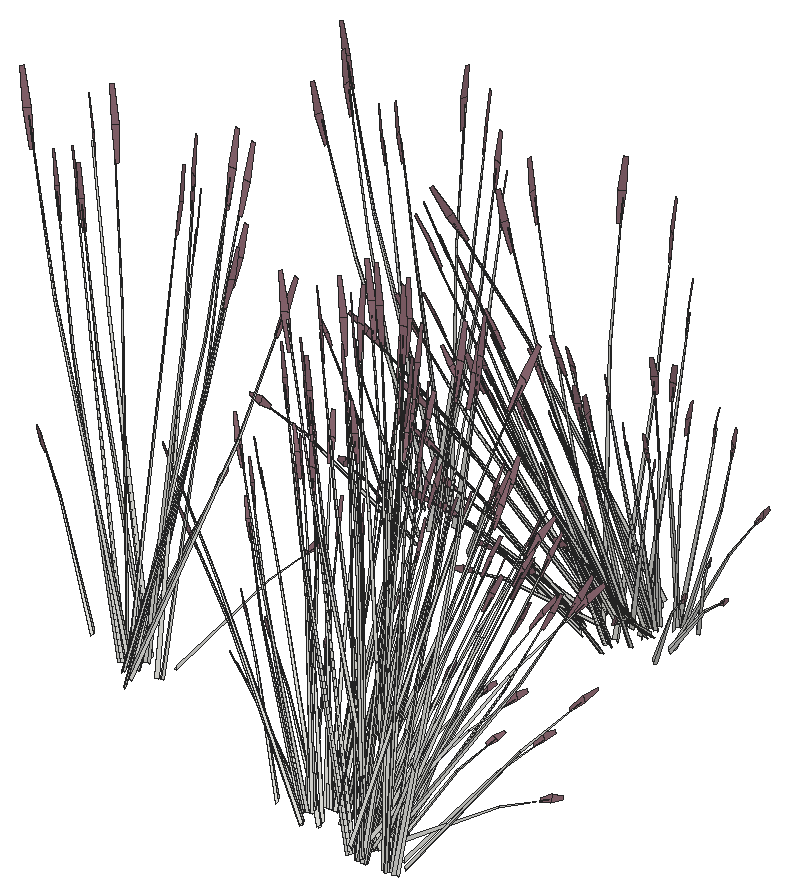
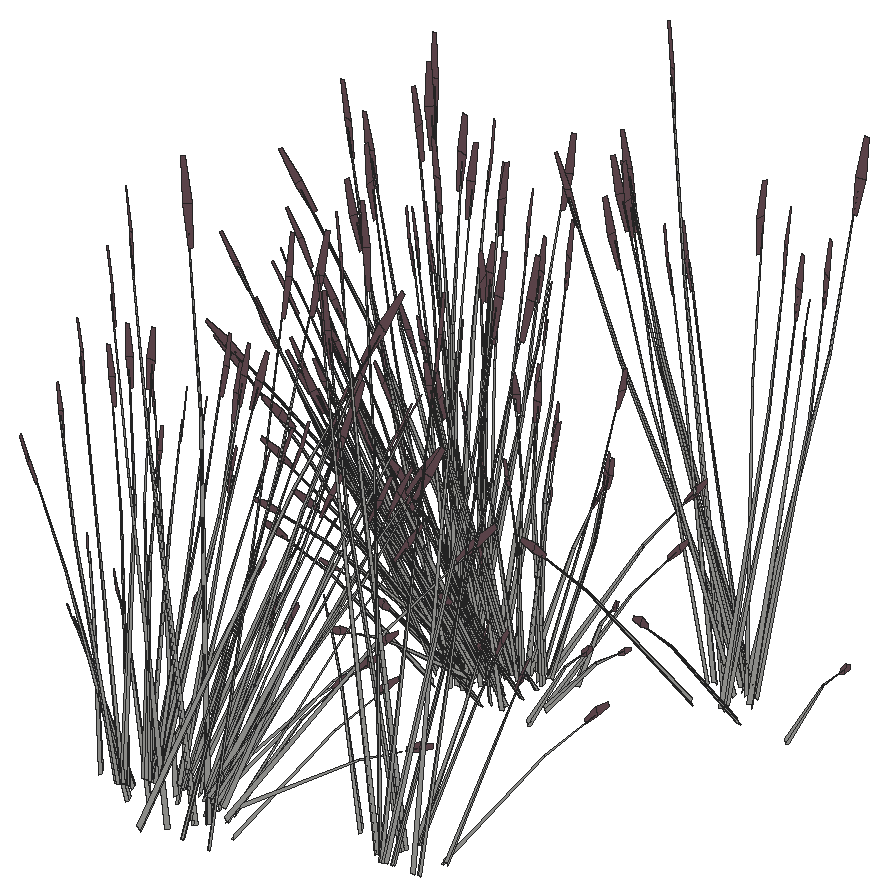
# SketchUp Ruby script. Lengths in inches.
U = 1.inch
M = Sketchup.active_model
def pt(a) = Geom::Point3d.new(a.map { |v| v * U })
def face(e, loops, mat)
  f = e.add_face(loops[0].map { |a| pt(a) })
  loops[1..].each { |l| e.add_face(l.map { |a| pt(a) }).erase! }
  f.material = f.back_material = mat if mat
  f
end
# faces: each face lists its corners as indices into pts; further lists are holes
def faces(e, pts, list, mat = nil) = list.each { |f| face(e, (f[0].is_a?(Array) ? f : [f]).map { |l| l.map { |i| pts[i] } }, mat) }
# xy, xz, yz: faces in a plane at the given z, y or x. An outline is a flat list of corners, or four numbers for a rectangle; further outlines are holes
def ring(l) = l.size == 4 ? [[l[0], l[1]], [l[2], l[1]], [l[2], l[3]], [l[0], l[3]]] : l.each_slice(2).to_a
def flat(e, list, mat, &to3) = list.each { |f| face(e, (f[0].is_a?(Array) ? f : [f]).map { |l| ring(l).map { |u, v| to3.(u, v) } }, mat) }
def xy(e, z, list, mat = nil) = flat(e, list, mat) { |x, y| [x, y, z] }
def xz(e, y, list, mat = nil) = flat(e, list, mat) { |x, z| [x, y, z] }
def yz(e, x, list, mat = nil) = flat(e, list, mat) { |y, z| [x, y, z] }
def lines(e, pts, list) = list.each { |a, b| e.add_line(pt(pts[a]), pt(pts[b])) }
# prism: a flat outline (further loops are holes) pulled along v
def prism(e, loops, v, mat = nil)
  f = face(e, loops, mat); d = Geom::Vector3d.new(v.map { |x| x * U })
  f.pushpull(f.normal.samedirection?(d) ? d.length : -d.length)
end
def box(e, o, s, mat = nil) = prism(e, [[o, [o[0] + s[0], o[1], o[2]], [o[0] + s[0], o[1] + s[1], o[2]], [o[0], o[1] + s[1], o[2]]]], [0, 0, s[2]], mat)
def at(x, y, z, deg = 0) = Geom::Transformation.translation(pt([x, y, z])) * Geom::Transformation.rotation(ORIGIN, Z_AXIS, deg.degrees)
def axes(o, x, y, z) = Geom::Transformation.new([*x, 0, *y, 0, *z, 0, *pt(o).to_a, 1])
def part(name) = M.definitions.add(name)
# library, detail: a bought-in or finely detailed component or shape, given as its bounding box
def library(name, o, s) = part(name).tap { |d| box(d.entities, o, s) }
def detail(e, o, s) = box(e.add_group.entities, o, s)
def put(e, d, t, mat = nil) = e.add_instance(d, t).tap { |i| i.material = mat if mat }
def group(e, t, mat = nil) = e.add_group.tap { |g| g.transformation = t; g.material = mat if mat }.entities
root = M.entities
M.materials.add("LightPink_Translucent").color = [144, 107, 117]
c1 = part("blade")
p = [[2.15,0.21,22],[0,0.17,0],[0.09,0.45,0],[2.18,0.31,22],[2.29,0.31,22],[0.38,0.45,0],
  [2.48,0.24,33],[2.49,0.24,33],[2.48,0.22,33]]
faces(c1.entities,p,[[0,1,2,3],[4,5,2,3],[6,3,4,7],[8,0,3,6]])
c2 = part("seeds")
p = [[0.3,-0.1,1.38],[-0.01,-0.03,1.59],[-0.01,-0.03,0.03],[0.14,-0.07,-0.07],[0.29,-0.03,3],[0.15,0.01,3.11]]
faces(c2.entities,p,[[0,1,2,3],[1,0,4,5]],"LightPink_Translucent")
c3 = part("blade with seeds")
put(c3.entities,c1,at(0,0,0))
put(c3.entities,c2,axes([2.4,0.25,30.99],[1.5799,-0.05474,1.17369],[-0.12525,1.92788,0.29478],[-0.07173,-0.02425,1.56792]))
put(root,c3,axes([79.25,512.875,37.29],[0.06562,-1.05324,-0.1216],[1.2424,0.02879,-0.67495],[0.4785,0.07316,1.02557]))
put(root,c3,axes([80.38,510.0625,34.73],[0,-1.03566,0.49651],[1.37109,0,0],[0,0.23588,1.57504]))
put(root,c3,axes([49.21,509.61,44.03],[0.28787,0.90242,-0.30978],[-1.14332,0.25625,0.30978],[0.23049,0.10406,1.38974]))
put(root,c3,axes([76.94,510.84,34.97],[1.33077,-0.06393,0.44739],[0.12035,1.06125,-0.21531],[-0.23824,0.10756,1.43643]))
put(root,c3,axes([77.77,509.76,34.87],[1.1418,-0.30203,0.1448],[0.39985,0.86246,-0.41347],[0,0.18981,1.26744]))
put(root,c3,axes([79.06,512.46,37.31],[-0.69728,-0.64842,0.35414],[0.79619,-0.61382,-0.4572],[0.40453,0.09339,0.87481]))
put(root,c3,axes([75.76,511.35,34.47],[-1.33077,0.06393,-0.44739],[-0.12035,-1.06125,0.21531],[-0.23824,0.10756,1.43643]))
put(root,c3,axes([82.02,511.86,34.85],[-0.29514,-0.25472,1.43002],[0.38401,-0.84262,-0.30754],[0.59714,0.11414,0.61141]))
put(root,c3,axes([47.17,514.54,44.18],[1.2866,-0.3514,-0.19198],[0.45209,1.01223,0.00008],[0.14202,-0.03884,1.73897]))
put(root,c3,axes([76.74,512.78,34.46],[1.23546,0.46496,0],[-0.59459,0.96613,0],[0,0,1.74954]))
put(root,c3,axes([47.86,511.2,44.06],[1.27479,0.1698,-0.62353],[-0.26901,1.04736,-0.16365],[0.38043,0.12691,1.37633]))
put(root,c3,axes([80.33,512.24,36.97],[0.26289,-0.01751,1.74944],[0.72108,-0.8046,-0.27667],[0.46761,0.10621,0.14031]))
put(root,c3,axes([77.23,513.8125,34.45],[-0.75665,-1.04141,-0.05142],[1.28187,-0.57875,0.51607],[-0.31588,0.09915,1.6363]))
put(root,c3,axes([76.97,511.29,34.87],[0.90538,0.62224,0.1448],[-0.75521,0.70202,-0.41347],[-0.21021,0.09491,1.26744]))
put(root,c3,axes([69.82,511.46,36.99],[-0.30393,-0.95317,0.48003],[1.19224,-0.16542,0.3958],[-0.35138,0.22417,0.9933]))
put(root,c3,axes([69.58,511.27,36.98],[-0.8413,-0.43556,0.0643],[0.48981,-0.62025,0.50621],[-0.26973,0.20053,0.77189]))
put(root,c3,axes([69.96,510.125,36.13],[0.42521,-0.21906,1.71376],[0.35798,1.01226,0.13857],[-0.66754,0.22878,0.73262]))
put(root,c3,axes([46.42,513.84,44.46],[-1.19666,-0.83357,-0.25192],[1.00694,-0.93603,0.5513],[-0.32224,0.09751,1.68216]))
put(root,c3,axes([79.31,512.37,37.24],[1.22504,0.02494,-0.71045],[-0.08228,1.05005,0.08574],[0.51899,0.11081,1.00501]))
put(root,c3,axes([77.93,513.21,34.73],[1.14694,-0.51783,0.49651],[0.68554,0.92854,0],[-0.26122,0.11794,1.57504]))
put(root,c3,axes([47.2,511.53,44.21],[0.73619,0.86927,-0.44739],[-1.11511,0.61213,0.21531],[0.23824,0.10756,1.43643]))
put(root,c3,axes([76.3,512.39,34.55],[0.53281,1.18979,-0.06012],[-1.52239,0.41691,0],[0.01861,0.04155,1.72173]))
put(root,c3,axes([76.89,513.68,34.28],[-1.14332,-0.25625,-0.30978],[0.28787,-0.90242,0.30978],[-0.23049,0.10406,1.38974]))
put(root,c3,axes([68.64,511.85,34.85],[0.42589,0.08502,1.43002],[0.2745,0.86839,-0.30754],[-0.57851,0.16255,0.61141]))
put(root,c3,axes([70.55,511.14,37.31],[1.06674,-0.14801,0.35414],[0.28168,0.84611,-0.4572],[-0.30569,0.22726,0.87481]))
put(root,c3,axes([81.31,510.24,34.63],[1.53239,0,0],[0,1.1575,-0.51607],[0,0.26363,1.63711]))
put(root,c3,axes([66.4375,510.76,36.96],[0.1564,0.02778,1.77383],[0.48382,0.91506,-0.16761],[-0.32016,0.24017,0.31391]))
put(root,c3,axes([80.7,510.83,34.45],[-1.53164,-0.00828,-0.04976],[0,-1.1575,0.49943],[-0.04813,0.2635,1.58352]))
put(root,c3,axes([77.38,509.83,34.92],[1.38012,0.49416,-0.29095],[-0.66454,1.04299,-0.50002],[0.04337,0.25608,1.59708]))
put(root,c3,axes([45.8125,513.66,44.21],[-1.33077,0.06393,-0.44739],[-0.12035,-1.06125,0.21531],[-0.23824,0.10756,1.43643]))
put(root,c3,axes([67.75,513.67,35.02],[0.51072,-0.46938,1.1486],[0.20153,0.74307,0.84392],[-0.36908,0.13305,0.25299]))
put(root,c3,axes([80.05,512.8,36.78],[0.69728,0.64842,-0.35414],[-0.79619,0.61382,0.4572],[0.40453,0.09339,0.87481]))
put(root,c3,axes([80.38,511,34.28],[-0.85545,0.64616,-0.30978],[-0.85545,-0.64616,0.30978],[0,0.20813,1.38974]))
put(root,c3,axes([76.69,511.06,34.92],[0.1428,1.18174,-0.29095],[-1.48733,0.07145,-0.50002],[-0.26191,0.15741,1.59708]))
put(root,c3,axes([79.6875,513.05,36.98],[-0.06171,0.78753,0.0643],[-0.9318,-0.02159,0.50621],[0.35694,0.08241,0.77189]))
put(root,c3,axes([77.24,510.6,34.47],[-0.59459,0.93321,-0.44739],[-1.23546,-0.44912,0.21531],[0,0.21512,1.43643]))
put(root,c3,axes([69.68,511.64,36.78],[-1.06674,0.14801,-0.35414],[-0.28168,-0.84611,0.4572],[-0.30569,0.22726,0.87481]))
put(root,c3,axes([79.77,512.8,36.99],[-0.90362,0.68241,0.48003],[-0.77932,-0.72471,0.3958],[0.42395,0.12588,0.9933]))
put(root,c3,axes([68.125,513.54,37.9],[1.08141,0.27645,-0.06488],[-0.33265,0.85086,-0.29416],[-0.17688,0.12919,0.97024]))
put(root,c3,axes([75.8,511.97,34.3125],[-0.82544,0.77843,-0.62353],[-1.0254,-0.70586,-0.16365],[-0.33076,0.19418,1.37633]))
put(root,c3,axes([76.9,513.59,37.31],[-0.18927,-0.83419,0.35414],[1.08199,-0.22027,-0.4572],[0.29062,0.23905,0.87481]))
put(root,c3,axes([77.27,513.28,34.58],[1.53422,0.33662,0.30756],[-0.38383,1.20322,-0.36492],[-0.25393,0.15059,1.64885]))
put(root,c3,axes([77.16,514.09,34.27],[-1.14694,0.51783,-0.49651],[-0.68554,-0.92854,0],[-0.26122,0.11794,1.57504]))
put(root,c3,axes([80.97,511.02,34.27],[0,1.03566,-0.49651],[-1.37109,0,0],[0,0.23588,1.57504]))
put(root,c3,axes([77.54,511.14,36.13],[-0.45521,-0.17844,1.71376],[0.94204,-0.74856,0.13857],[0.58713,0.33769,0.73262]))
put(root,c3,axes([77.63,508.79,36.73],[-1.05895,-0.53811,1.38283],[1.11816,-0.83781,0.59665],[0.34166,0.5049,1.33663]))
put(root,c3,axes([70,511.0625,37.29],[1.1336,0.57106,-0.1216],[-0.65308,0.827,-0.67495],[-0.32027,0.28747,1.02557]))
put(root,c3,axes([46.94,515.99,44.03],[-1.14332,-0.25625,-0.30978],[0.28787,-0.90242,0.30978],[-0.23049,0.10406,1.38974]))
put(root,c3,axes([79.23,513.17,35.02],[-0.69001,-0.29779,1.1486],[0.89096,-0.30257,0.84392],[0.24031,0.2563,0.25299]))
put(root,c3,axes([76.8,514.02,37.29],[0.73026,-0.88648,-0.1216],[1.05755,0.51071,-0.67495],[0.36761,0.25045,1.02557]))
put(root,c3,axes([71.52,510.81,36.13],[0.30609,-0.31822,1.71376],[0.77286,0.85893,0.13857],[-0.53009,0.39116,0.73262]))
put(root,c3,axes([47.4375,512.13,44.67],[1.38012,0.49416,-0.29095],[-0.66454,1.04299,-0.50002],[0.04337,0.25608,1.59708]))
put(root,c3,axes([70.56,511.74,36.94],[0.31482,0.94565,-0.51099],[-1.19224,0.16542,-0.3958],[-0.34166,0.254,0.97773]))
put(root,c3,axes([50.43,513.31,44.03],[-0.85545,0.64616,-0.30978],[-0.85545,-0.64616,0.30978],[0,0.20813,1.38974]))
put(root,c3,axes([71.99,512.83,37.31],[0.82919,-0.54528,0.35414],[0.78493,0.62262,-0.4572],[-0.11943,0.31634,0.87481]))
put(root,c3,axes([78.2,513.93,34.63],[0.7662,1.03778,0],[-1.28187,0.57875,-0.51607],[-0.29196,0.13181,1.63711]))
put(root,c3,axes([46.75,513.37,44.67],[0.1428,1.18174,-0.29095],[-1.48733,0.07145,-0.50002],[-0.26191,0.15741,1.59708]))
put(root,c3,axes([75.85,514.76,36.96],[0.00363,-0.12539,1.77383],[1.0502,-0.55319,-0.16761],[0.36479,0.19745,0.31391]))
put(root,c3,axes([47.29,512.91,44.21],[-0.59459,0.93321,-0.44739],[-1.23546,-0.44912,0.21531],[0,0.21512,1.43643]))
put(root,c3,axes([79.42,514.28,33.75],[0.08928,-0.14952,1.76342],[1.12407,-0.44035,-0.26939],[0.34078,0.22791,0.30037]))
put(root,c3,axes([77.55,509.82,35.1],[-0.03348,-0.97511,1.41272],[1.51511,0.25277,0.59816],[-0.35835,0.53357,1.3335]))
put(root,c3,axes([77.94,510.88,34.35],[0.44936,0.94823,-0.69212],[-1.29441,0.3415,-0.18165],[0.04967,0.32109,1.52773]))
put(root,c3,axes([71.24,513.32,36.98],[-1.00708,-0.04826,0.0643],[0.02761,-0.72867,0.50621],[-0.10538,0.27912,0.77189]))
put(root,c3,axes([69.1,514.15,33.75],[0.16438,0.10347,1.76342],[0.27873,0.95868,-0.26939],[-0.36432,0.20444,0.30037]))
put(root,c3,axes([71.56,513.39,36.99],[-0.87265,-0.70663,0.48003],[0.92674,-0.60943,0.3958],[-0.16097,0.33153,0.9933]))
put(root,c3,axes([77.67,513.58,36.94],[1.20928,-0.24619,-0.51099],[0.21154,0.93233,-0.3958],[0.32481,0.26718,0.97773]))
put(root,c3,axes([74.3125,513.72,37.31],[0.36946,-0.79643,0.35414],[1.07787,0.23229,-0.4572],[0.09883,0.32066,0.87481]))
put(root,c3,axes([45.85,514.27,44.06],[-0.82544,0.77843,-0.62353],[-1.0254,-0.70586,-0.16365],[-0.33076,0.19418,1.37633]))
put(root,c3,axes([79.34,514.53,34.92],[-0.78586,-0.03248,1.0506],[0.51898,-0.68985,0.58006],[0.31045,0.24509,0.8241]))
put(root,c3,axes([77.07,514.35,36.98],[-0.55698,0.6579,0.0643],[-0.79316,-0.38303,0.50621],[0.25643,0.21093,0.77189]))
put(root,c3,axes([47.21,516.4,44.02],[-1.14694,0.51783,-0.49651],[-0.68554,-0.92854,0],[-0.26122,0.11794,1.57504]))
put(root,c3,axes([51.02,513.33,44.02],[0,1.03566,-0.49651],[-1.37109,0,0],[0,0.23588,1.57504]))
put(root,c3,axes([75.76,516.5625,37.9],[0.84686,-0.59414,-0.06488],[0.77596,0.65071,-0.29416],[0.05463,0.18438,0.97024]))
put(root,c3,axes([77.31,514.16,36.99],[-1.21888,0.23767,0.48003],[-0.21154,-0.93233,0.3958],[0.28666,0.27478,0.9933]))
put(root,c3,axes([71.29,511.59,36.13],[0.22818,-0.35597,1.71376],[0.95725,0.73667,0.13857],[-0.43183,0.45914,0.73262]))
put(root,c3,axes([76.77,512.86,34.85],[0.02163,-0.34331,1.43002],[1.03345,-0.38348,-0.30754],[0.31903,0.4109,0.61141]))
put(root,c3,axes([73.98,514.44,36.98],[-0.90301,0.35198,0.0643],[-0.44199,-0.64184,0.50621],[0.08721,0.28293,0.77189]))
put(root,c3,axes([71.55,513.6,36.78],[-0.82919,0.54528,-0.35414],[-0.78493,-0.62262,0.4572],[-0.11943,0.31634,0.87481]))
put(root,c3,axes([68.7,513.4375,36.97],[-0.03046,0.20495,1.74944],[0.86449,0.71297,-0.27667],[-0.22632,0.33716,0.14031]))
put(root,c3,axes([71.46,512.98,37.65],[1.34686,0.05131,-0.13498],[-0.03681,0.97156,-0.74919],[-0.09356,0.37418,1.13838]))
put(root,c3,axes([73.95,514.06,37.29],[1.19922,-0.48218,-0.1216],[0.58932,0.85579,-0.67495],[0.15822,0.36063,1.02557]))
put(root,c3,axes([74.3,514.38,37.32],[-1.20755,-0.27075,0.53283],[0.41292,-0.89013,0.43934],[0.07257,0.35005,1.10256]))
put(root,c3,axes([72.08,515.72,35.02],[-0.03171,-0.6158,1.1486],[0.7925,0.43922,0.84392],[-0.15586,0.29352,0.25299]))
put(root,c3,axes([49.47,516.59,43.49],[0.08928,-0.14952,1.76342],[1.12407,-0.44035,-0.26939],[0.34078,0.22791,0.30037]))
put(root,c3,axes([47.99,513.19,44.09],[0.44936,0.94823,-0.69212],[-1.29441,0.3415,-0.18165],[0.04967,0.32109,1.52773]))
put(root,c3,axes([39.15,516.46,43.49],[0.16438,0.10347,1.76342],[0.27873,0.95868,-0.26939],[-0.36432,0.20444,0.30037]))
put(root,c3,axes([74.17,514.25,33.75],[0.19833,-0.05635,1.76342],[1.19302,0.31018,-0.26939],[0.03489,0.3496,0.30037]))
put(root,c3,axes([72.38,513.34,37.26],[0.87728,0.69587,-0.5672],[-0.92674,0.60943,-0.43934],[-0.13348,0.35356,1.08528]))
put(root,c3,axes([71.43,514.39,35.08],[1.11329,-0.1834,0.06507],[0.25594,0.73887,-0.86304],[-0.07058,0.37403,0.7736]))
put(root,c3,axes([74.98,514.02,36.94],[1.20468,0.25962,-0.51099],[-0.41292,0.89013,-0.3958],[0.11046,0.35838,0.97773]))
put(root,c3,axes([75.66,512.18,36.13],[-0.28013,-0.33252,1.71376],[1.29445,-0.27994,0.13857],[0.29256,0.52202,0.73262]))
put(root,c3,axes([74.43,514.5625,36.78],[-0.36946,0.79643,-0.35414],[-1.07787,-0.23229,0.4572],[0.09883,0.32066,0.87481]))
put(root,c3,axes([72.11,513.02,37.59],[-0.03189,0.95798,-0.7886],[-1.34277,-0.06434,0.09517],[-0.14171,0.40585,1.11556]))
put(root,c3,axes([68.6,515.54,36.96],[0.13903,-0.06253,1.77383],[1.14912,0.41591,-0.16761],[-0.027,0.34629,0.31391]))
put(root,c3,axes([73.38,512.34,36.13],[-0.02999,-0.3975,1.71376],[1.30002,0.26369,0.13857],[-0.08041,0.56647,0.73262]))
put(root,c3,axes([74.54,513.85,37.24],[0.5849,0.8421,-0.71045],[-1.20401,0.4693,0.08574],[0.13677,0.40688,1.00501]))
put(root,c3,axes([71.16,515.17,34.85],[0.38672,-0.16338,1.43002],[0.95481,0.49262,-0.30754],[-0.28419,0.42626,0.61141]))
put(root,c3,axes([44.22,516.55,43.49],[0.19833,-0.05635,1.76342],[1.19302,0.31018,-0.26939],[0.03489,0.3496,0.30037]))
put(root,c3,axes([73.67,515.97,36.97],[0.15534,0.16677,1.74944],[1.25362,0.06552,-0.27667],[0.12606,0.3678,0.14031]))
put(root,c3,axes([71.66,514.37,35.62],[0.02693,-0.53464,1.54345],[1.21102,0.2824,0.21329],[-0.10493,0.5698,0.72882]))
put(root,c3,axes([53.05,550.03,43.49],[-0.20555,0.03731,1.76342],[-1.13672,-0.42002,-0.26939],[0.01907,-0.35034,0.30037]))
put(root,c3,axes([72.59,552.82,41.15],[0.28013,0.33252,1.71376],[-1.29445,0.27994,0.13857],[-0.29256,-0.52202,0.73262]))
put(root,c3,axes([74.73,550.61,41.99],[-0.18744,-0.14521,1.74944],[-1.25089,0.09206,-0.27667],[-0.19964,-0.34731,0.14031]))
put(root,c3,axes([77.625,552.34,39.87],[-0.34835,0.20963,1.43002],[-1.04325,-0.36691,-0.30754],[0.19338,-0.4563,0.61141]))
put(root,c3,axes([76.04,553.07,42.26],[-0.5849,-0.8421,-0.71045],[1.20401,-0.4693,0.08574],[-0.13677,-0.40688,1.00501]))
put(root,c3,axes([72.23,551.9375,39.87],[-0.07421,0.33879,1.43002],[-1.08488,0.28361,-0.30754],[-0.25359,-0.4379,0.61141]))
put(root,c3,axes([75.03,551.2,38.77],[-0.20555,0.03731,1.76342],[-1.13672,-0.42002,-0.26939],[0.01907,-0.35034,0.30037]))
put(root,c3,axes([78.47,553.89,42.26],[0.03189,-0.95798,-0.71045],[1.34277,0.06434,0.08574],[0.14171,-0.40585,1.00501]))
put(root,c3,axes([80.35,552.39,41.99],[-0.01183,-0.20612,1.74944],[-0.99913,-0.59572,-0.27667],[0.15447,-0.36112,0.14031]))
put(root,c3,axes([76.15,552.35,41.8],[0.36946,-0.79643,-0.35414],[1.07787,0.23229,0.4572],[-0.09883,-0.32066,0.87481]))
put(root,c3,axes([76.96,553.4,41.15],[-0.22818,0.35597,1.71376],[-0.95725,-0.73667,0.13857],[0.43183,-0.45914,0.73262]))
put(root,c3,axes([80.08,551.65,41.99],[-0.12446,0.07911,1.77383],[-1.21937,-0.26689,-0.16761],[-0.04414,-0.34521,0.31391]))
put(root,c3,axes([75.6,552.9,41.96],[-1.20468,-0.25962,-0.51099],[0.41292,-0.89013,-0.3958],[-0.11046,-0.35838,0.97773]))
put(root,c3,axes([76.34,550.67,40.04],[0.15721,0.60392,1.1486],[-0.87211,-0.33448,0.84392],[0.09385,-0.30923,0.25299]))
put(root,c3,axes([78.2,553.57,41.96],[-0.87728,-0.69587,-0.51099],[0.92674,-0.60943,-0.3958],[0.13348,-0.35356,0.97773]))
put(root,c3,axes([73.44,550.14,41.99],[-0.02286,0.12414,1.77383],[-1.12758,0.45052,-0.16761],[-0.33182,-0.23029,0.31391]))
put(root,c3,axes([73.2,552.34,42.37],[1.36515,-0.26619,0.53763],[0.23692,1.04421,0.4433],[-0.32106,-0.30775,1.11249]))
put(root,c3,axes([49.375,551.3125,43.49],[-0.11871,0.13643,1.76342],[-1.19964,0.29415,-0.26939],[-0.2898,-0.26759,0.30037]))
put(root,c3,axes([76.28,552.53,42.01],[1.20755,0.27075,0.48003],[-0.41292,0.89013,0.3958],[-0.07257,-0.35005,0.9933]))
put(root,c3,axes([76.63,552.85,42.3125],[-1.19922,0.48218,-0.1216],[-0.58932,-0.85579,-0.67495],[-0.15822,-0.36063,1.02557]))
put(root,c3,axes([79.12,553.9375,42.3125],[-1.34686,-0.05131,-0.1216],[0.03681,-0.97156,-0.67495],[0.09356,-0.37418,1.02557]))
put(root,c3,axes([79.03,553.3125,41.8],[0.82919,-0.54528,-0.35414],[0.78493,0.62262,0.4572],[0.11943,-0.31634,0.87481]))
put(root,c3,axes([51.35,555.0625,44.1],[-0.50328,-1.06202,-0.69835],[1.44974,-0.38248,-0.18329],[-0.05563,-0.35963,1.54149]))
put(root,c3,axes([71.86,551.39,40.04],[0.63926,0.36046,1.1486],[-0.93099,0.21668,0.84392],[-0.1992,-0.27702,0.25299]))
put(root,c3,axes([76.6,552.47,42.01],[0.90301,-0.35198,0.0643],[0.44199,0.64184,0.50621],[-0.08721,-0.28293,0.77189]))
put(root,c3,axes([73.4,553.3,42.26],[-1.04497,-0.50058,-0.71045],[0.74264,-0.8772,0.08574],[-0.3786,-0.29889,1.00501]))
put(root,c3,axes([58.08,551.82,43.49],[-0.18342,-0.08159,1.76342],[-0.47115,-0.9115,-0.26939],[0.31784,-0.24736,0.30037]))
put(root,c3,axes([73.04,552.64,41.8],[-0.18927,-0.83419,-0.35414],[1.08199,-0.22027,0.4572],[-0.29062,-0.23905,0.87481]))
put(root,c3,axes([73.51,552.57,42.01],[0.55698,-0.6579,0.0643],[0.79316,0.38303,0.50621],[-0.25643,-0.21093,0.77189]))
put(root,c3,axes([71.35,552.48,38.77],[-0.11871,0.13643,1.76342],[-1.19964,0.29415,-0.26939],[-0.2898,-0.26759,0.30037]))
put(root,c3,axes([73.33,556.23,39.375],[-0.50328,-1.06202,-0.69835],[1.44974,-0.38248,-0.18329],[-0.05563,-0.35963,1.54149]))
put(root,c3,axes([52.84,550.76,44.13],[-0.84686,0.59414,-0.03893],[-0.77596,-0.65071,-0.17649],[-0.05463,-0.18438,0.58215]))
put(root,c3,axes([70.71,553.85,41.15],[0.45521,0.17844,1.71376],[-0.94204,0.74856,0.13857],[-0.58713,-0.33769,0.73262]))
put(root,c3,axes([80.0625,552.98,38.77],[-0.18342,-0.08159,1.76342],[-0.47115,-0.9115,-0.26939],[0.31784,-0.24736,0.30037]))
put(root,c3,axes([76.27,553.1875,42.33],[-0.36946,0.79643,0.35414],[-1.07787,-0.23229,-0.4572],[-0.09883,-0.32066,0.87481]))
put(root,c3,axes([72.91,553.33,41.96],[-1.20928,0.24619,-0.51099],[-0.21154,-0.93233,-0.3958],[-0.32481,-0.26718,0.97773]))
put(root,c3,axes([79.02,553.53,42.01],[0.87265,0.70663,0.48003],[-0.92674,0.60943,0.3958],[0.16097,-0.33153,0.9933]))
put(root,c3,axes([73.76,552.5,42.71],[-0.81789,0.99285,-0.13619],[-1.18445,-0.572,-0.75594],[-0.41173,-0.28051,1.14864]))
put(root,c3,axes([79.35,553.59,42.01],[1.00708,0.04826,0.0643],[-0.02761,0.72867,0.50621],[0.10538,-0.27912,0.77189]))
put(root,c3,axes([78.59,554.09,42.33],[-0.82919,0.54528,0.35414],[-0.78493,-0.62262,-0.4572],[0.11943,-0.31634,0.87481]))
put(root,c3,axes([80.06,555.55,42.26],[0.64013,-0.81717,-0.71045],[1.12174,0.58074,0.08574],[0.38221,-0.29607,1.00501]))
put(root,c3,axes([48.39,554.91,44.02],[0,-1.03566,-0.49651],[1.37109,0,0],[0,-0.23588,1.57504]))
put(root,c3,axes([52.2,551.85,44.02],[1.14694,-0.51783,-0.49651],[0.68554,0.92854,0],[0.26122,-0.11794,1.57504]))
put(root,c3,axes([73.14,553.17,39.65],[-0.7662,-1.03778,0],[1.28187,-0.57875,-0.51607],[0.29196,-0.13181,1.63711]))
put(root,c3,axes([80.02,555.17,41.96],[-0.31482,-0.94565,-0.51099],[1.19224,-0.16542,-0.3958],[0.34166,-0.254,0.97773]))
put(root,c3,axes([74.82,551.92,39.41],[-0.84686,0.59414,-0.03893],[-0.77596,-0.65071,-0.17649],[-0.05463,-0.18438,0.58215]))
put(root,c3,axes([53.56,553.97,44.06],[0.82544,-0.77843,-0.62353],[1.0254,0.70586,-0.16365],[0.33076,-0.19418,1.37633]))
put(root,c3,axes([70.625,552.21,41.99],[-0.26368,-0.00731,1.74944],[-0.83946,0.73103,-0.27667],[-0.44791,-0.14937,0.14031]))
put(root,c3,axes([80.59,555.85,42.3125],[-1.1336,-0.57106,-0.1216],[0.65308,-0.827,-0.67495],[0.32027,-0.28747,1.02557]))
put(root,c3,axes([75.9,558.97,40.6],[1.05902,0.41762,1.51261],[-1.03748,0.89969,0.59816],[-0.46471,-0.53324,1.26806]))
put(root,c3,axes([52.12,555.34,44.21],[0.59459,-0.93321,-0.44739],[1.23546,0.44912,0.21531],[0,-0.21512,1.43643]))
put(root,c3,axes([73.68,553.32,42.33],[0.18927,0.83419,0.35414],[-1.08199,0.22027,-0.4572],[-0.29062,-0.23905,0.87481]))
put(root,c3,axes([52.66,554.875,44.67],[-0.1428,-1.18174,-0.29095],[1.48733,-0.07145,-0.50002],[0.26191,-0.15741,1.59708]))
put(root,c3,axes([70.37,556.08,39.3],[0,-1.03566,-0.49651],[1.37109,0,0],[0,-0.23588,1.57504]))
put(root,c3,axes([74.18,553.01,39.3],[1.14694,-0.51783,-0.49651],[0.68554,0.92854,0],[0.26122,-0.11794,1.57504]))
put(root,c3,axes([48.98,554.9375,44.03],[0.85545,-0.64616,-0.30978],[0.85545,0.64616,0.30978],[0,-0.20813,1.38974]))
put(root,c3,axes([80.98,554.8,39.87],[-0.4378,-0.03068,1.43002],[-0.44851,-0.8229,-0.30754],[0.53783,-0.23279,0.61141]))
put(root,c3,axes([70.43,553.86,42.37],[1.01205,-0.7643,0.53763],[0.87284,0.81167,0.4433],[-0.47482,-0.14098,1.11249]))
put(root,c3,axes([83.38,555.6,41.99],[-0.16006,-0.00787,1.77383],[-0.66468,-0.8428,-0.16761],[0.26693,-0.27711,0.31391]))
put(root,c3,axes([48.63,551.84,44.13],[-0.35352,0.84566,-0.03893],[-1.08806,-0.26014,-0.17649],[-0.1652,-0.13832,0.58215]))
put(root,c3,axes([51.97,556.11,44.67],[-1.38012,-0.49416,-0.29095],[0.66454,-1.04299,-0.50002],[-0.04337,-0.25608,1.59708]))
put(root,c3,axes([75.54,555.14,39.34],[0.82544,-0.77843,-0.62353],[1.0254,0.70586,-0.16365],[0.33076,-0.19418,1.37633]))
put(root,c3,axes([81.49,553.29,40.04],[-0.40819,0.5272,1.1486],[-0.35086,-0.70831,0.84392],[0.33713,-0.17749,0.25299]))
put(root,c3,axes([52.47,552.26,44.03],[1.14332,0.25625,-0.30978],[-0.28787,0.90242,0.30978],[0.23049,-0.10406,1.38974]))
put(root,c3,axes([80.9,555.27,41.8],[1.06674,-0.14801,-0.35414],[0.28168,0.84611,0.4572],[0.30569,-0.22726,0.87481]))
